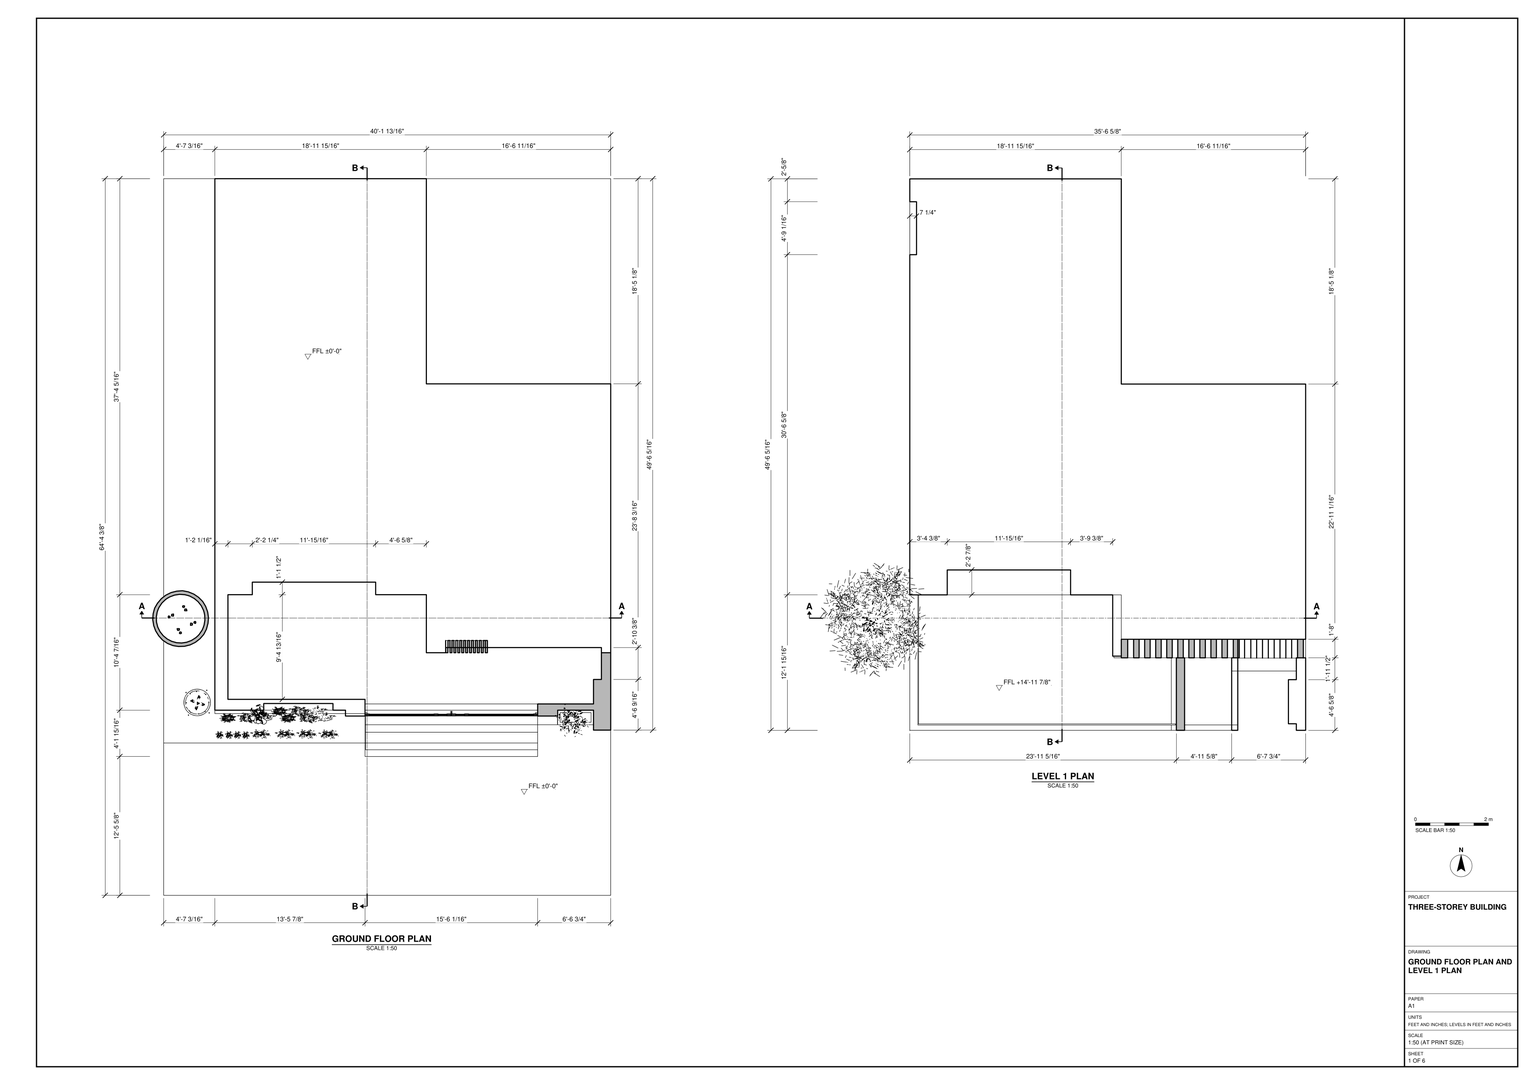
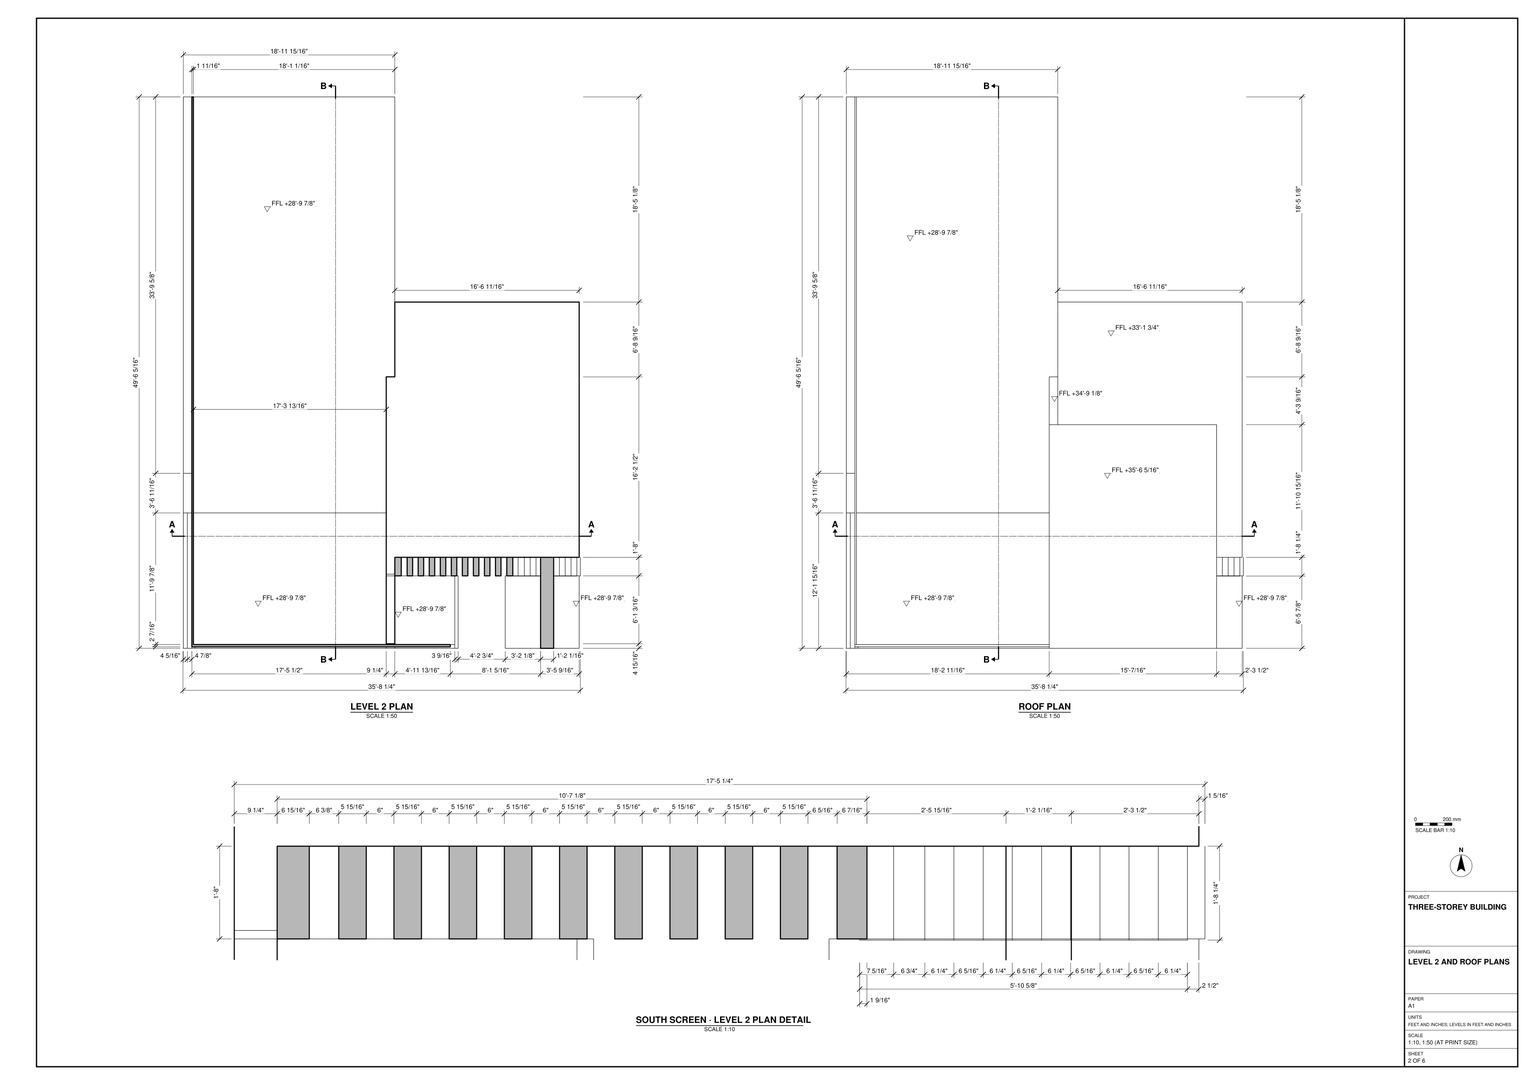
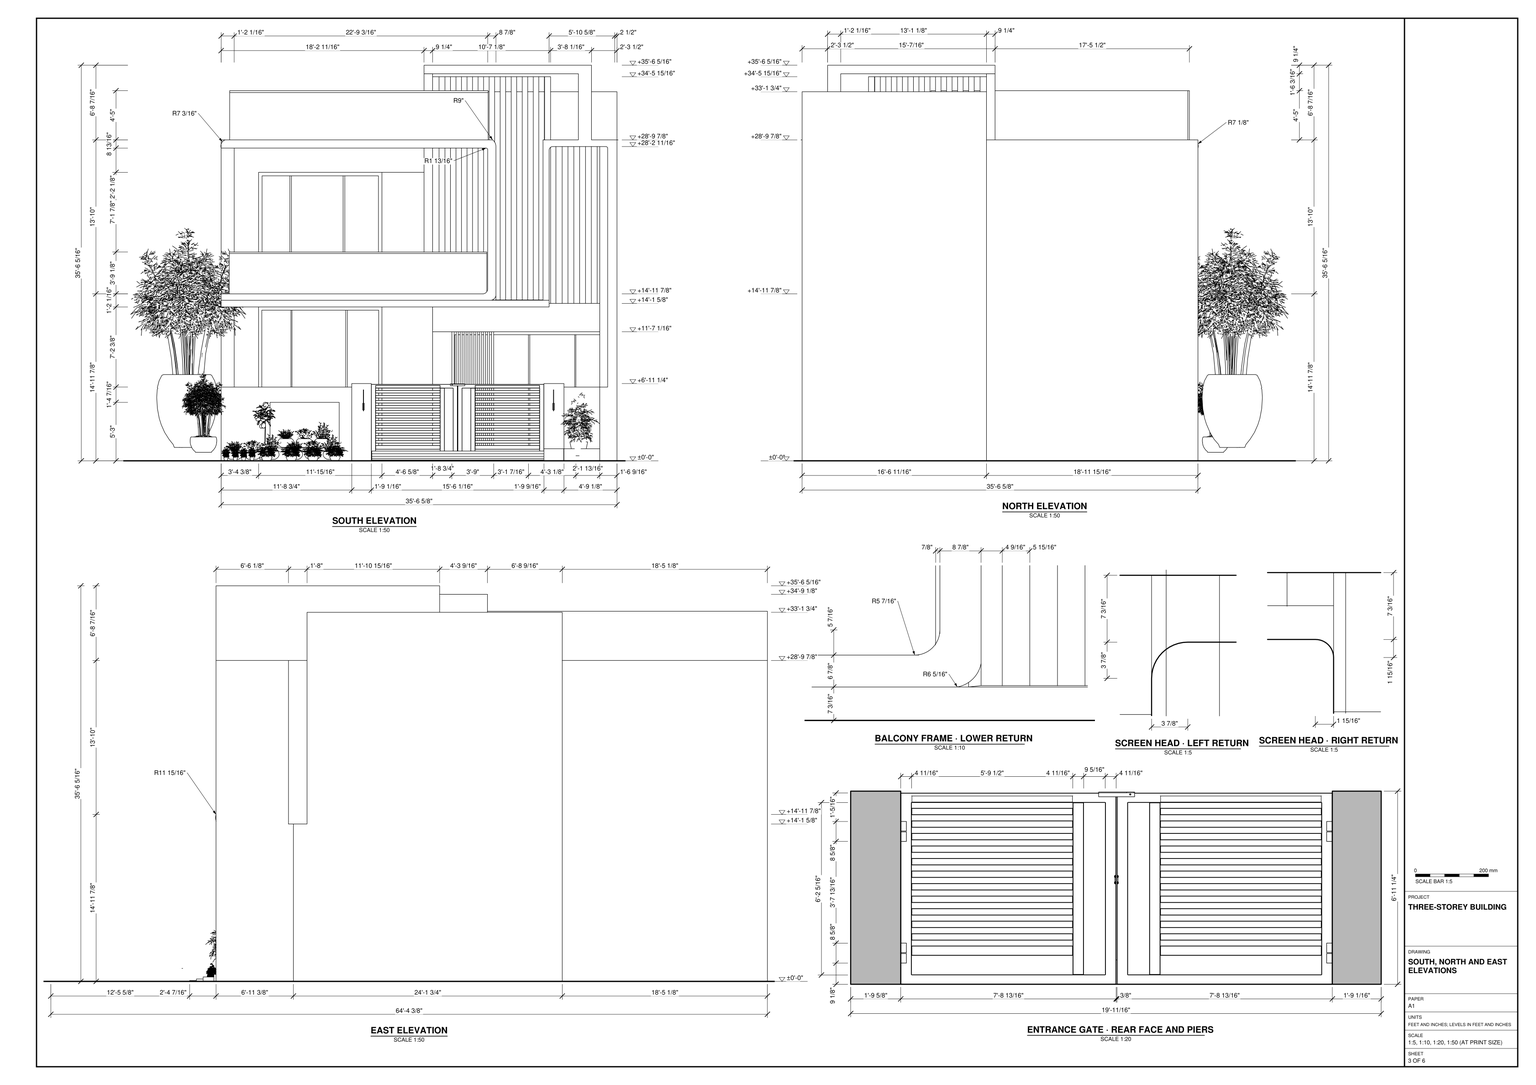
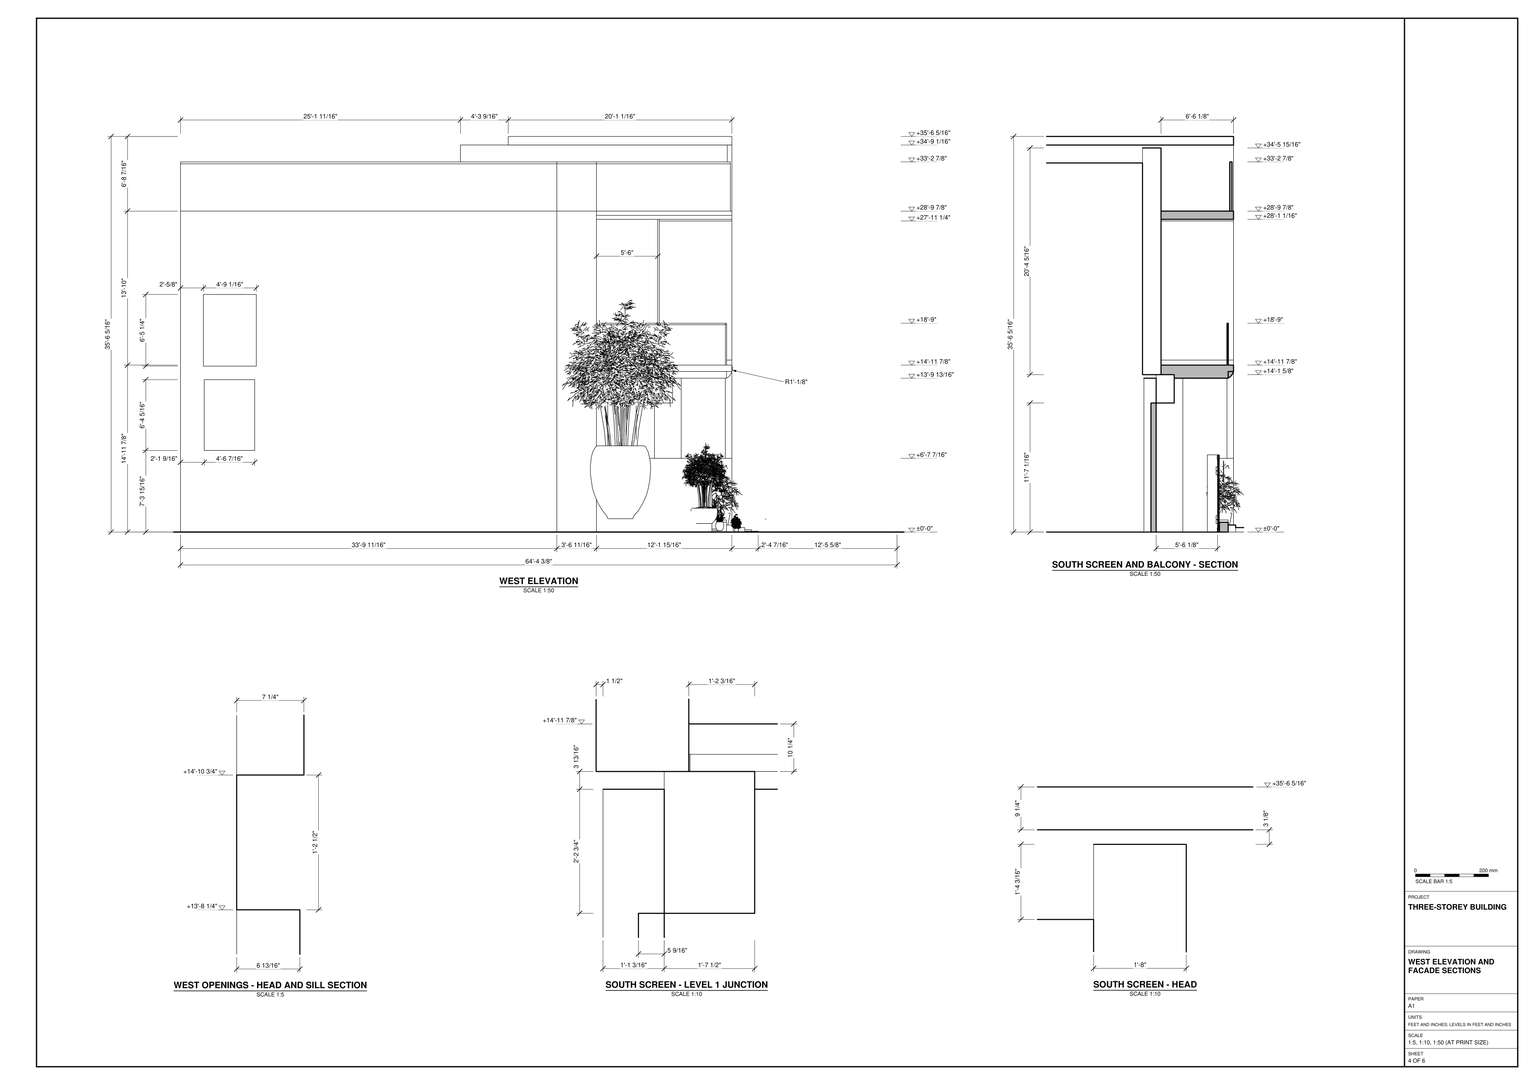
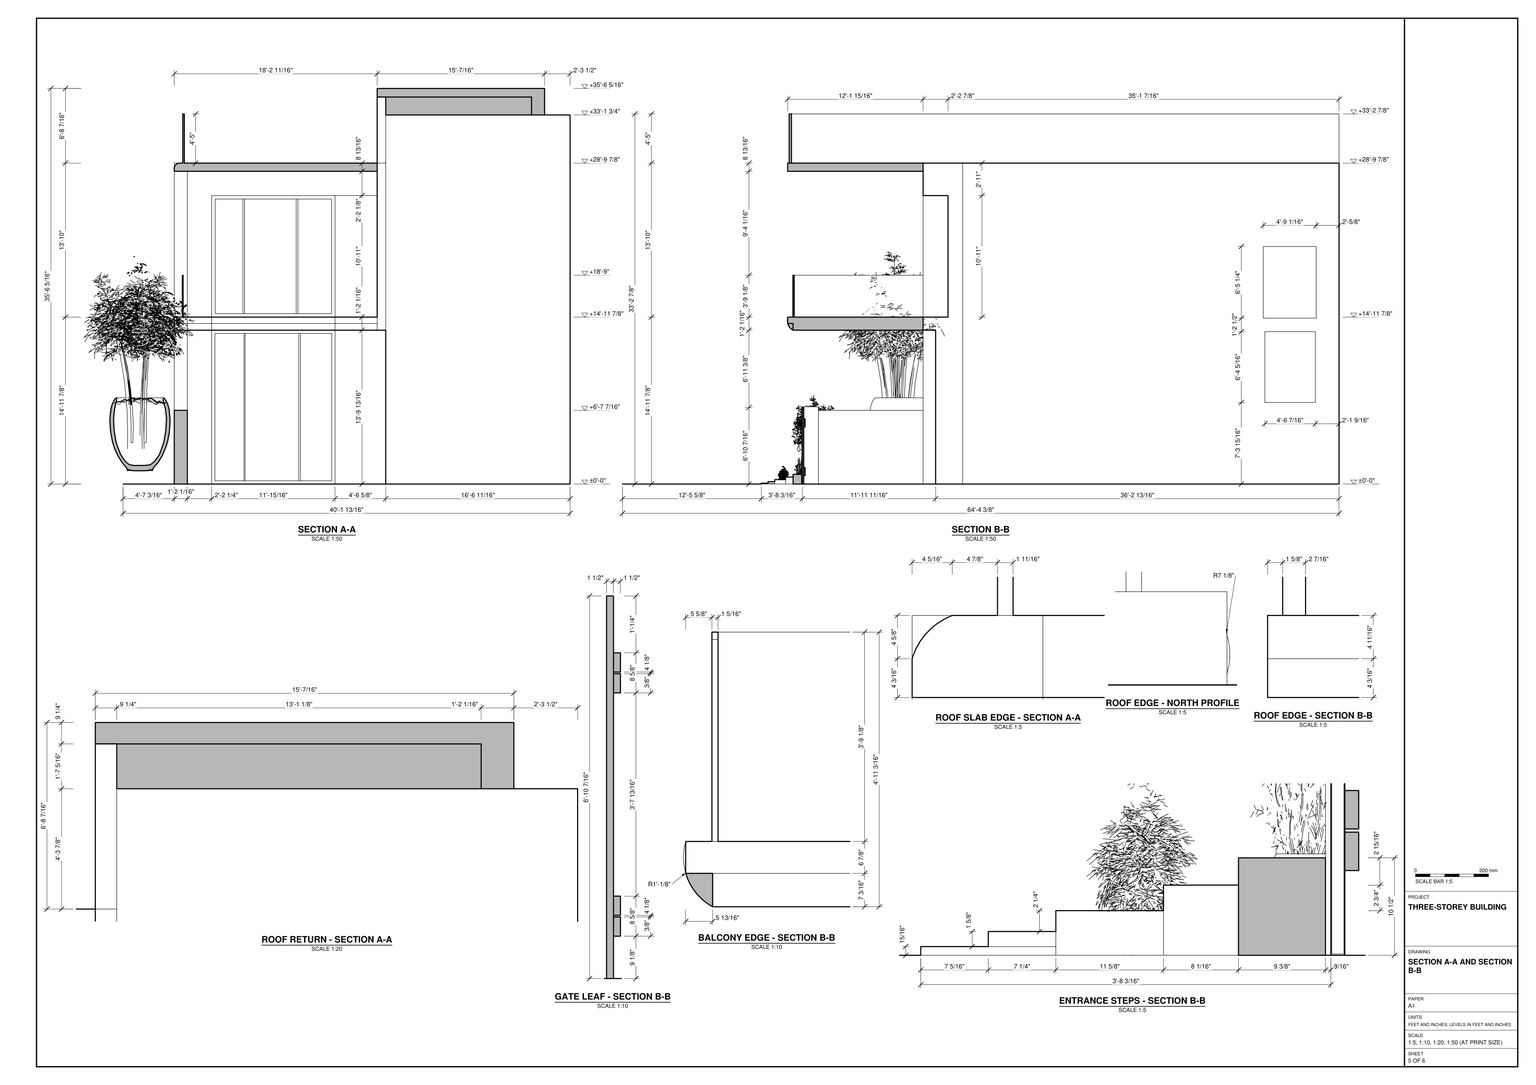
Build the three-storey building and its entrance frontage in SketchUp using task_files/diagram_01.pdf. Work in feet and inches. The complete model shall measure 43'-9 1/8" along X, 64'-4 3/8" along Y and 35'-6 5/16" along Z. Set the ground floor at ±0'-0", Level 1 at +14'-11 7/8" and Level 2 at +28'-9 7/8".

Follow the plans for the stepped footprint, wall thicknesses, openings and slab edges. Use the roof plan and elevations together to locate the changes in roof height. On the south elevation, set the upper glazing behind the balcony parapet, form the rounded returns of the projecting balcony frame, and carry the vertical screen fins up to the raised roof frame. Model the lower glazing, entrance steps, gate leaves and piers, using the rear-face detail for the gate. Include the planting in the positions shown on the frontage plan. Decor and loose items, including plants and lights, may use any suitable library components.

Keep shell elements such as walls, slabs and roof separate as groups or components. Do the same for each furniture or joinery piece shown, and use components for repeated parts such as screen fins. Save one SketchUp model as output_files/three_storey_building_with_a_screened_south_balcony.skp.

# SketchUp Ruby script. Lengths in inches.
U = 1.inch
M = Sketchup.active_model
def pt(a) = Geom::Point3d.new(a.map { |v| v * U })
def face(e, loops, mat)
  f = e.add_face(loops[0].map { |a| pt(a) })
  loops[1..].each { |l| e.add_face(l.map { |a| pt(a) }).erase! }
  f.material = f.back_material = mat if mat
  f
end
# faces: each face lists its corners as indices into pts; further lists are holes
def faces(e, pts, list, mat = nil) = list.each { |f| face(e, (f[0].is_a?(Array) ? f : [f]).map { |l| l.map { |i| pts[i] } }, mat) }
# xy, xz, yz: faces in a plane at the given z, y or x. An outline is a flat list of corners, or four numbers for a rectangle; further outlines are holes
def ring(l) = l.size == 4 ? [[l[0], l[1]], [l[2], l[1]], [l[2], l[3]], [l[0], l[3]]] : l.each_slice(2).to_a
def flat(e, list, mat, &to3) = list.each { |f| face(e, (f[0].is_a?(Array) ? f : [f]).map { |l| ring(l).map { |u, v| to3.(u, v) } }, mat) }
def xy(e, z, list, mat = nil) = flat(e, list, mat) { |x, y| [x, y, z] }
def xz(e, y, list, mat = nil) = flat(e, list, mat) { |x, z| [x, y, z] }
def yz(e, x, list, mat = nil) = flat(e, list, mat) { |y, z| [x, y, z] }
def lines(e, pts, list) = list.each { |a, b| e.add_line(pt(pts[a]), pt(pts[b])) }
# prism: a flat outline (further loops are holes) pulled along v
def prism(e, loops, v, mat = nil)
  f = face(e, loops, mat); d = Geom::Vector3d.new(v.map { |x| x * U })
  f.pushpull(f.normal.samedirection?(d) ? d.length : -d.length)
end
def box(e, o, s, mat = nil) = prism(e, [[o, [o[0] + s[0], o[1], o[2]], [o[0] + s[0], o[1] + s[1], o[2]], [o[0], o[1] + s[1], o[2]]]], [0, 0, s[2]], mat)
def at(x, y, z, deg = 0) = Geom::Transformation.translation(pt([x, y, z])) * Geom::Transformation.rotation(ORIGIN, Z_AXIS, deg.degrees)
def axes(o, x, y, z) = Geom::Transformation.new([*x, 0, *y, 0, *z, 0, *pt(o).to_a, 1])
def part(name) = M.definitions.add(name)
# library, detail: a bought-in or finely detailed component or shape, given as its bounding box
def library(name, o, s) = part(name).tap { |d| box(d.entities, o, s) }
def detail(e, o, s) = box(e.add_group.entities, o, s)
def put(e, d, t, mat = nil) = e.add_instance(d, t).tap { |i| i.material = mat if mat }
def group(e, t, mat = nil) = e.add_group.tap { |g| g.transformation = t; g.material = mat if mat }.entities
root = M.entities
M.materials.add("Material__11").color = [91, 133, 74]
M.materials.add("Material__3").color = [47, 40, 35]
M.materials.add("Material__4").color = [45, 34, 22]
M.materials.add("Material__6").color = [53, 66, 30]
M.materials.add("Niraj_Hair_Dark").color = [109, 109, 109]
M.materials.add("Niraj_Shirt").color = [144, 153, 181]
M.materials.add("[0129_WhiteSmoke]").color = [245, 245, 245]
M.materials.add("[0130_Gainsboro]").color = [220, 220, 220]
M.materials.add("[Asphalt New]").color = [67, 60, 62]
M.materials.add("[Basic Tile]").color = [203, 206, 202]
M.materials.add("[Cladding Siding Tan]").color = [162, 126, 95]
M.materials.add("[Field Square Tile]").color = [217, 201, 169]
M.materials.add("[Grass Dark Green]").color = [106, 157, 55]
M.materials.add("[Translucent Glass Gray]").color = [128, 128, 128]
M.materials["[Translucent Glass Gray]"].alpha = 0.5
M.materials.add("[Wood Floor Parquet]").color = [145, 89, 39]
M.materials.add("[Wood Veneer 01]").color = [120, 70, 37]
M.materials.add("bronze").color = [85, 58, 39]
M.materials.add("light bulb").color = [254, 239, 217]
M.materials.add("wire_1").color = [17, 17, 17]
c1 = library("Slatted double gate",[7.03,-128.55,-3.91],[5.33,99.02,60.06])
c2 = part("Linear wall light")
g1 = group(c2.entities,at(0.6875,0,0.79))
xy(g1,0,[[0,0,0.39,8.27],[[0,8.27,0.39,22.83],[0.04,8.31,0.35,22.8]]])
xy(g1,0.04,[[0.04,8.31,0.35,22.8]],"light bulb")
xy(g1,0.39,[[0,0,0.39,22.83]])
xz(g1,0,[[0,0,0.39,0.39]])
xz(g1,8.31,[[0.04,0,0.35,0.04]])
xz(g1,22.8,[[0.04,0,0.35,0.04]])
xz(g1,22.83,[[0,0,0.39,0.39]])
yz(g1,0,[[0,0,22.83,0.39]])
yz(g1,0.04,[[8.31,0,22.8,0.04]])
yz(g1,0.35,[[8.31,0,22.8,0.04]])
yz(g1,0.39,[[0,0,22.83,0.39]])
g2 = group(c2.entities,at(0,1.18,0))
box(g2,[0,0,0],[1.77,7.09,0.79])
c3 = part("WALL+LIGHT+50")
put(c3.entities,c2,axes([4.75,-2.61,16.86],[1,0,0],[0,0,1],[0,-1,0]),"bronze")
put(c3.entities,c2,axes([209.625,-2.61,16.86],[1,0,0],[0,0,1],[0,-1,0]),"bronze")
c4 = library("plants",[0.18,-0.67,0.63],[15.85,6.49,10.81])
c5 = library("Group\#17",[-156.07,-132.78,403.82],[328.27,343.15,49.73])
c6 = library("Group\#15",[-190.47,-156.43,0],[392.44,392.43,450])
c7 = library("Group\#18",[-224.63,-110.83,370.48],[360.75,278.69,1335.95])
c8 = library("Group\#19",[-170.17,-135.75,412.97],[353.33,352.63,31.3])
c9 = library("Group\#14",[-390.42,-321.9,981.25],[712.69,695.89,825.3])
c10 = part("Potted tree")
p = [[391.42,322.9,0],[390.42,321.9,0],[391.42,321.9,0]]
lines(c10.entities,p,[[0,1],[1,2],[2,0]])
put(c10.entities,c5,at(390.42,321.9,0),"Material__3")
put(c10.entities,c6,at(390.42,321.9,0))
put(c10.entities,c7,at(390.42,321.9,0),"Material__4")
g3 = group(c10.entities,at(390.42,321.9,0),"wire_1")
xy(g3,2.45,[[-59.6,-46.28,-36.375,-34.93,-11.68,-29.34,15.46,-33.14,46.57,-25.27,76.1,-6.18,100.39,22.24,98.66,53.87,95.77,65.28,88.08,79.53,87.97,84.15,87.1,85.66,83.13,88.01,74.2,100.3,66.09,109.96,37.49,121.54,1.58,115.97,-27.44,104.75,-47.08,82.45,-56.52,55.13,-74.46,34.57,-97.22,27.4375,-113.62,-7.42,-100.95,-13.99,-91.64,-16.18,-96.41,-18.55,-93.97,-22.4375,-89.59,-19.73,-91.56,-27.7,-91.98,-39.95]],"wire_1")
put(c10.entities,c8,at(390.42,321.9,0),"Material__3")
put(c10.entities,c9,at(390.42,321.9,0),"Material__6")
c11 = library("Group\#24",[-51.25,-16.26,0.11],[32.43,32.44,25.32])
c12 = library("Group\#29",[-68.4,-38.23,21.61],[71.82,69.27,94.54])
c13 = library("Group\#31",[0,0,0],[126.13,128.05,229.04])
c14 = library("Group\#32",[0,23.8125,0],[126.13,128.06,238.18])
c15 = part("BAMBOO+PLANTS+18")
p = [[0,0,0],[1,0,0],[1,1,0]]
lines(c15.entities,p,[[0,1],[1,2],[2,0]])
put(c15.entities,c11,axes([-463.4375,32.99,-14],[0.36589,0,0],[0,0.16797,0],[0,0,0.16797]))
put(c15.entities,c12,axes([-463.4375,32.99,-14],[0.36589,0,0],[0,0.16797,0],[0,0,0.16797]),"Material__11")
put(c15.entities,c13,axes([-568.04,42.06,-4.9],[0.38,0,0],[0,0.38,0],[0,0,0.38]))
put(c15.entities,c11,axes([-119.36,48.1875,-8.59],[0.59,0,0],[0,0.59,0],[0,0,0.59]))
put(c15.entities,c12,axes([-119.36,48.1875,-8.59],[0.59,0,0],[0,0.59,0],[0,0,0.59]),"Material__11")
put(c15.entities,c14,at(-623.98,68,0.35))
put(c15.entities,c11,axes([-436.93,32.99,-14],[0.36589,0,0],[0,0.16797,0],[0,0,0.16797]))
put(c15.entities,c12,axes([-436.93,32.99,-14],[0.36589,0,0],[0,0.16797,0],[0,0,0.16797]),"Material__11")
put(c15.entities,c12,axes([-413.65,32.99,-14],[0.36589,0,0],[0,0.16797,0],[0,0,0.16797]),"Material__11")
put(c15.entities,c11,axes([-413.65,32.99,-14],[0.36589,0,0],[0,0.16797,0],[0,0,0.16797]))
put(c15.entities,c11,axes([-390,32.72,-13.61],[0.36589,0,0],[0,0.16797,0],[0,0,0.16797]))
put(c15.entities,c12,axes([-390,32.72,-13.61],[0.36589,0,0],[0,0.16797,0],[0,0,0.16797]),"Material__11")
put(c15.entities,c12,axes([-505.28,31.89,-14],[0.14036,0,0],[0,0.14036,0],[0,0,0.14036]),"Material__11")
put(c15.entities,c11,axes([-487.28,31.66,-13.67],[0.14036,0,0],[0,0.14036,0],[0,0,0.14036]))
put(c15.entities,c12,axes([-487.28,31.66,-13.67],[0.14036,0,0],[0,0.14036,0],[0,0,0.14036]),"Material__11")
put(c15.entities,c11,axes([-505.28,31.89,-14],[0.14036,0,0],[0,0.14036,0],[0,0,0.14036]))
put(c15.entities,c11,axes([-515.45,31.89,-14],[0.14036,0,0],[0,0.14036,0],[0,0,0.14036]))
put(c15.entities,c12,axes([-515.45,31.89,-14],[0.14036,0,0],[0,0.14036,0],[0,0,0.14036]),"Material__11")
put(c15.entities,c11,axes([-496.35,31.89,-14],[0.14036,0,0],[0,0.14036,0],[0,0,0.14036]))
put(c15.entities,c12,axes([-496.35,31.89,-14],[0.14036,0,0],[0,0.14036,0],[0,0,0.14036]),"Material__11")
c16 = library("Group\#2",[0,0,0],[149.58,6.3125,301.125])
c17 = library("Group\#3",[0,0,0],[149.58,6.3125,301.125])
c18 = library("Group\#1",[0,0,0],[78.59,6.3125,301.125])
xy(root,0,[[463.28,178.07,481.82,178.07,481.82,261.48,471.78,261.48,471.78,232.66,463.28,232.66,463.28,206.28,403.07,206.28,403.07,193.25,424.67,193.25,424.67,199.56,463.28,199.56],[217.61,183.87,424.39,193.25],[424.39,183.87,424.67,193.25],[[424.67,183.87,463.28,199.56],[427.29,186.49,460.66,196.9375]],[427.29,186.49,460.66,196.9375],
  [217.61,193.25,403.07,193.25,403.07,199.56,217.02,199.56,217.02,195.87,217.61,195.87],[55.17,195.87,195.95,199.56],[217.02,199.56,403.07,206.28],[217.02,206.28,463.28,206.28,463.28,232.66,471.78,232.66,471.78,267.04,303.9,267.04,303.9,261.48,283.13,261.48,283.13,324.02,228.49,324.02,228.49,337.52,95.53,337.52,95.53,324.02,69.26,324.02,69.26,211.22,217.02,211.22],[283.13,551.23,481.82,772.36]])
xy(root,0,[[0,0,481.82,0,481.82,178.07,463.28,178.07,463.28,183.87,403.07,183.87,403.07,149.62,217.02,149.62,217.02,164.18,0,164.18]],"[Basic Tile]")
xy(root,0,[[195.95,193.25,217.02,195.87],[195.95,195.87,217.02,195.87,217.02,211.22,69.26,211.22,69.26,324.02,95.53,324.02,95.53,337.52,228.49,337.52,228.49,324.02,283.13,324.02,283.13,261.48,303.9,261.48,303.9,267.04,471.78,267.04,471.78,261.48,481.82,261.48,481.82,551.23,283.13,551.23,283.13,772.36,55.17,772.36,55.17,199.56,195.95,199.56]],"[Field Square Tile]")
xy(root,0,[[0,164.18,217.02,164.18,217.02,193.25,195.95,193.25,195.95,195.87,55.17,195.87,55.17,772.36,0,772.36],[217.02,164.18,217.61,183.87],[217.02,183.87,217.61,193.25],[217.02,193.25,217.61,195.87]],"[Grass Dark Green]")
xy(root,0.9375,[[217.02,149.62,403.07,149.62,403.07,156.9,217.61,156.9,217.61,164.18,217.02,164.18]],"[Field Square Tile]")
xy(root,2.5625,[[217.61,156.9,403.07,164.18]],"[Field Square Tile]")
xy(root,4.8125,[[217.61,164.18,403.07,175.79]],"[Field Square Tile]")
xy(root,7.5625,[[217.61,175.79,403.07,183.87]],"[Field Square Tile]")
xy(root,10.5,[[217.61,183.87,403.07,193.25]],"[Field Square Tile]")
xy(root,13,[[403.07,183.87,424.39,193.25],[[424.67,183.87,463.28,199.56],[427.29,186.49,460.66,196.9375]]],"[Asphalt New]")
xy(root,13.87,[[107.84,199.56,182.46,206.75]])
xy(root,62.99,[[107.84,199.56,182.46,206.75]])
xy(root,79.4375,[[463.28,178.07,471.78,185.12],[463.28,185.12,471.78,199.56],[55.17,199.56,195.95,199.56,195.95,211.22,69.26,211.22,69.26,324.02,55.17,324.02],[424.67,199.56,458.84,199.56,458.84,203.37,463.28,203.37,463.28,206.28,424.67,206.28],[458.84,199.56,463.28,203.37]])
xy(root,83.25,[[195.95,193.25,217.02,211.22],[403.07,193.25,424.67,206.28]])
xy(root,87.94,[[55.17,692.36,61.99,746.8]],"[0129_WhiteSmoke]")
xy(root,139.07,[[465.71,241.98,471.78,267.04]])
xy(root,139.07,[[283.13,241.98,303.9,261.48],[303.9,241.98,465.71,267.04]],"[Asphalt New]")
xy(root,164.25,[[55.17,692.36,61.99,746.8]],"[0129_WhiteSmoke]")
xy(root,165.8125,[[95.53,324.02,228.49,337.52]])
xy(root,165.8125,[[55.17,183.87,55.17,324.02,283.13,324.02,283.13,241.98,408.69,241.98,408.69,183.87]],"[Field Square Tile]")
xy(root,169.64,[[283.13,241.98,351.34,256.18],[408.69,241.98,471.78,241.98,471.78,256.18,481.82,256.18,481.82,276.16,283.13,276.16,283.13,256.18,408.69,256.18],[351.34,241.98,408.69,256.18]])
xy(root,173.02,[[55.17,178.06,346.23,178.07],[55.17,178.07,346.23,183.87],[346.23,178.07,348.65,183.87],[348.65,178.07,408.69,183.87],[346.23,183.87,348.65,197.12],
  [275.14,224.23,283.13,256.18]])
xy(root,173.33,[[351.34,178.07,402.09,256.18]])
xy(root,178.78,[[55.17,690.64,62.42,747.7]],"[0129_WhiteSmoke]")
xy(root,179.89,[[55.17,178.06,337.03,178.06,337.03,183.71,63.89,183.71,63.89,324.02,55.17,324.02],[337.03,183.71,341.53,185.04],[64.7,185.04,337.03,185.04,337.03,256.18,275.14,256.18,275.14,258,273.88,258,273.88,324.02,64.7,324.02],[275.14,256.18,283.13,258],[95.53,324.02,228.49,350.9]])
xy(root,225.02,[[63.89,183.71,341.53,185.04],[63.89,185.04,64.7,324.02]],"Niraj_Hair_Dark")
xy(root,256.03,[[55.17,690.64,62.42,747.7]],"[0129_WhiteSmoke]")
xy(root,310.89,[[95.53,324.02,228.49,350.9]])
xy(root,337.03,[[273.88,256.18,283.13,258]])
xy(root,337.03,[[55.17,178.06,55.17,324.02,69.26,324.02,69.26,206.96,340.65,206.96,340.65,178.06]],"[Field Square Tile]")
xy(root,337.03,[[69.26,206.96,256.26,324.02],[256.26,206.96,256.26,324.02,273.88,324.02,273.88,256.18,340.65,256.18,340.65,206.96]],"[Wood Floor Parquet]")
xy(root,338.67,[[412.59,178.07,469.83,185.12]])
xy(root,342.31,[[463.28,185.12,471.78,232.66]])
xy(root,345.875,[[59.49,178.06,64.375,324.02],[64.375,178.06,67.74,179.68],[67.74,178.06,273.88,179.68],[273.88,178.06,283.13,179.68],[283.13,178.06,347.76,178.06,347.76,182.15,342.94,182.15,342.94,179.68,283.13,179.68],
  [64.375,179.68,342.94,182.15],[66.05,182.15,273.88,324.02],[273.88,182.15,283.13,183],[283.13,182.15,347.76,256.18],[273.88,183,283.13,256.18],
  [64.375,324.02,66.05,772.36],[66.05,324.02,273.88,324.02,273.88,470.65,283.13,470.65,283.13,772.36,66.05,772.36],[55.17,366.7,64.375,772.36]])
xy(root,345.875,[[55.17,324.02,64.375,366.7]],"Niraj_Shirt")
xy(root,345.875,[[402.09,178.07,440.24,256.18],[454.32,178.07,481.82,256.18],[440.24,256.18,454.32,276.16]],"[0129_WhiteSmoke]")
xy(root,397.75,[[283.13,276.16,440.24,276.16,440.24,419.1,454.32,419.1,454.32,276.16,481.82,276.16,481.82,551.23,283.13,551.23]])
xy(root,397.75,[[440.24,276.16,454.32,419.1]],"[0129_WhiteSmoke]")
xy(root,398.875,[[64.375,179.68,342.94,182.15],[64.375,182.15,66.05,772.36]],"Niraj_Hair_Dark")
xy(root,417.08,[[283.13,178.07,283.13,183,273.88,183,273.88,419.1,440.24,419.1,440.24,178.07]],"[0129_WhiteSmoke]")
xy(root,417.125,[[273.88,178.07,283.13,183],[273.88,183,283.13,470.65]])
xy(root,426.3125,[[273.88,178.07,454.32,419.1]],"[0129_WhiteSmoke]")
xz(root,149.62,[[217.02,0,403.07,0.9375]],"[Field Square Tile]")
xz(root,156.9,[[217.61,0.9375,403.07,2.5625]],"[Field Square Tile]")
xz(root,164.18,[[217.02,0,217.61,0.9375]])
xz(root,164.18,[[217.61,2.5625,403.07,4.8125]],"[Field Square Tile]")
xz(root,175.79,[[217.61,4.8125,403.07,7.5625]],"[Field Square Tile]")
xz(root,178.06,[[55.17,173.02,346.23,173.02,346.85,173.16,347.46,173.37,348.04,173.64,348.59,173.97,348.65,174.01,349.11,174.35,349.58,174.78,350.01,175.25,350.39,175.77,350.71,176.32,350.98,176.9,351.19,177.5,351.34,178.125,351.34,338.7,351.3125,339.39,351.23,340.08,351.1,340.76,350.92,341.43,350.68,342.08,350.4,342.71,350.0625,343.32,349.68,343.9,349.26,344.44,348.8,344.96,348.3,345.4375,347.76,345.875,59.49,345.875,58.67,345.5,57.9,345.03,57.2,344.46,56.58,343.8125,56.04,343.09,55.59,342.31,55.25,341.47,55.17,341.21,55.17,337.03,340.65,337.03,340.89,337.02,341.12,336.97,341.34,336.9,341.56,336.79,341.75,336.66,341.93,336.5,342.09,336.33,342.22,336.13,342.32,335.92,342.4,335.69,342.45,335.46,342.46,335.23,342.46,185.33,342.41,184.62,342.28,183.92,342.05,183.25,341.73,182.61,341.34,182.02,340.87,181.48,340.33,181.01,339.74,180.62,339.11,180.31,338.43,180.08,337.74,179.9375,337.03,179.89,55.17,179.89],[55.17,337.03,55.17,341.21,55.01,340.6,54.88,339.71,54.87,338.81,54.96,337.91]])
xz(root,178.07,[[463.28,0,481.82,0,481.82,345.875,454.32,345.875,454.32,426.3125,273.88,426.3125,273.88,417.125,283.13,417.125,283.13,417.08,440.24,417.08,440.24,345.875,402.09,345.875,402.09,173.33,351.34,173.33,348.65,173.02,408.69,173.02,408.69,334.77,408.73,335.28,408.83,335.78,408.99,336.26,409.22,336.72,409.5,337.14,409.83,337.53,410.22,337.86,410.64,338.15,411.1,338.37,411.58,338.54,412.08,338.64,412.59,338.67,469.83,338.67,470.08,338.65,470.33,338.6,470.57,338.52,470.8,338.41,471.01,338.27,471.21,338.1,471.375,337.91,471.52,337.69,471.63,337.47,471.71,337.22,471.76,336.97,471.78,336.72,471.78,79.4375,463.28,79.4375]])
xz(root,179.68,[[64.375,396.83,342.94,398.875]],"Niraj_Hair_Dark")
xz(root,179.68,[[64.375,345.875,342.94,396.83]],"[Translucent Glass Gray]")
xz(root,182.15,[[66.05,345.875,342.94,398.875]],"[Translucent Glass Gray]")
xz(root,183,[[273.88,345.875,283.13,417.08],[273.88,417.08,283.13,417.125]])
xz(root,183.71,[[63.89,223.42,341.53,225.02]],"Niraj_Hair_Dark")
xz(root,183.71,[[63.89,179.89,341.53,223.42]],"[Translucent Glass Gray]")
xz(root,183.87,[[217.61,0,403.07,7.5625],[55.17,165.8125,408.69,173.02]])
xz(root,183.87,[[403.07,0,424.39,13],[424.67,0,463.28,13]],"[Asphalt New]")
xz(root,183.87,[[217.61,7.5625,403.07,10.5]],"[Field Square Tile]")
xz(root,185.04,[[63.89,179.89,64.7,225.02]])
xz(root,185.04,[[64.7,179.89,341.53,225.02]],"[Translucent Glass Gray]")
xz(root,185.12,[[463.28,79.4375,471.78,79.4375,471.78,336.72,471.76,336.97,471.71,337.22,471.63,337.47,471.52,337.69,471.375,337.91,471.21,338.1,471.01,338.27,470.8,338.41,470.57,338.52,470.33,338.6,470.08,338.65,469.83,338.67,463.28,338.67],[471.78,336.72,471.78,342.31,463.28,342.31,463.28,338.67,469.83,338.67,470.08,338.65,470.33,338.6,470.57,338.52,470.8,338.41,471.01,338.27,471.21,338.1,471.375,337.91,471.52,337.69,471.63,337.47,471.71,337.22,471.76,336.97]])
xz(root,186.49,[[427.29,0,460.66,13]])
xz(root,193.25,[[195.95,0,217.02,83.25],[217.61,0,403.07,10.5],[403.07,0,424.39,13],[424.39,0,424.67,0,424.67,83.25,403.07,83.25,403.07,13,424.39,13]])
xz(root,196.9375,[[427.29,0,460.66,13]],"[Asphalt New]")
xz(root,197.12,[[346.23,173.02,348.65,173.02,348.65,174.01,348.59,173.97,348.04,173.64,347.46,173.37,346.85,173.16],[348.65,173.02,351.34,173.02,351.34,173.33],[348.65,173.02,351.34,173.33,351.34,178.125,351.19,177.5,350.98,176.9,350.71,176.32,350.39,175.77,350.01,175.25,349.58,174.78,349.11,174.35,348.65,174.01],[348.65,174.01,349.11,174.35,349.58,174.78,350.01,175.25,350.39,175.77,350.71,176.32,350.98,176.9,351.19,177.5,351.34,178.125,348.65,178.125]])
xz(root,199.56,[[[55.17,0,195.95,79.4375],[107.84,13.87,182.46,62.99]],[424.67,0,463.28,13],[424.67,13,463.28,79.4375]])
xz(root,206.28,[[403.07,0,403.07,83.25,424.67,83.25,424.67,79.4375,463.28,79.4375,463.28,0]])
xz(root,206.75,[[107.84,13.87,182.46,62.99]])
xz(root,211.22,[[69.26,0,217.02,79.4375],[195.95,79.4375,217.02,83.25]])
xz(root,232.66,[[463.28,0,471.78,342.31]])
xz(root,241.98,[[283.13,165.8125,408.69,169.64]])
xz(root,241.98,[[283.13,139.07,471.78,139.07,471.78,169.64,408.69,169.64,408.69,165.8125,283.13,165.8125]],"[Asphalt New]")
xz(root,256.18,[[283.13,169.64,283.13,179.89,342.46,179.89,342.46,337.03,283.13,337.03,283.13,345.875,347.76,345.875,348.3,345.4375,348.8,344.96,349.26,344.44,349.68,343.9,350.0625,343.32,350.4,342.71,350.68,342.08,350.92,341.43,351.1,340.76,351.23,340.08,351.3125,339.39,351.34,338.7,351.34,169.64],[351.34,169.64,351.34,173.33,402.09,173.33,402.09,330.87,408.69,330.87,408.69,169.64],[471.78,169.64,481.82,330.87],[275.14,173.02,283.13,179.89],[337.03,179.89,337.74,179.9375,338.43,180.08,339.11,180.31,339.74,180.62,340.33,181.01,340.87,181.48,341.34,182.02,341.73,182.61,342.05,183.25,342.28,183.92,342.41,184.62,342.46,185.33,342.46,179.89],
  [471.78,330.87,481.82,345.875],[342.46,335.23,342.45,335.46,342.4,335.69,342.32,335.92,342.22,336.13,342.09,336.33,341.93,336.5,341.75,336.66,341.56,336.79,341.34,336.9,341.12,336.97,340.89,337.02,340.65,337.03,342.46,337.03],[273.88,337.03,283.13,345.875]])
xz(root,256.18,[[402.09,330.87,408.69,345.875]],"[0129_WhiteSmoke]")
xz(root,258,[[273.88,179.89,283.13,337.03]])
xz(root,261.48,[[471.78,0,481.82,139.07]])
xz(root,261.48,[[283.13,0,303.9,139.07]],"[Asphalt New]")
xz(root,267.04,[[303.9,0,386.39,0,386.39,3.15,307.06,3.15,307.06,135.91,468.625,135.91,468.625,3.15,387.84,3.15,387.84,0,471.78,0,471.78,139.07,303.9,139.07],[386.39,0,387.84,3.15],[386.39,3.15,387.84,135.91],[436.29,3.15,437.49,135.91]],"[Asphalt New]")
xz(root,267.04,[[307.06,3.15,386.39,135.91],[387.84,3.15,436.29,135.91],[437.49,3.15,468.625,135.91]],"[Translucent Glass Gray]")
xz(root,276.16,[[440.24,345.875,454.32,397.75]],"[0129_WhiteSmoke]")
xz(root,276.16,[[410.27,345.875,440.24,397.75],[454.32,345.875,481.82,397.75]],"[Translucent Glass Gray]")
xz(root,276.16,[[283.13,169.64,481.82,169.64,481.82,345.875,410.27,345.875,410.27,397.75,283.13,397.75]],"[Wood Floor Parquet]")
xz(root,324.02,[[55.17,165.8125,69.26,173.02],[69.26,165.8125,95.53,173.02],[95.53,165.8125,228.49,173.02],[228.49,165.8125,273.88,173.02],[55.17,173.02,55.17,179.89,63.89,179.89,63.89,225.02,64.7,225.02,64.7,179.89,69.26,179.89,69.26,173.02],
  [69.26,173.02,95.53,179.89],[95.53,173.02,228.49,179.89],[228.49,173.02,273.88,179.89],[55.17,337.03,55.17,341.21,55.25,341.47,55.59,342.31,56.04,343.09,56.58,343.8125,57.2,344.46,57.9,345.03,58.67,345.5,59.49,345.875,69.26,345.875,69.26,337.03],[69.26,337.03,95.53,345.875],
  [95.53,337.03,228.49,345.875],[228.49,337.03,273.88,345.875],[55.17,341.21,55.17,345.875,59.49,345.875,58.67,345.5,57.9,345.03,57.2,344.46,56.58,343.8125,56.04,343.09,55.59,342.31,55.25,341.47]])
xz(root,324.02,[[55.17,79.4375,69.26,165.8125],[55.17,179.89,63.89,179.89,63.89,225.02,64.7,225.02,64.7,179.89,69.26,179.89,69.26,337.03,55.17,337.03]],"Niraj_Shirt")
xz(root,324.02,[[69.26,0,95.53,165.8125],[69.26,179.89,95.53,179.89,95.53,310.89,273.88,310.89,273.88,337.03,69.26,337.03]],"[Asphalt New]")
xz(root,324.02,[[228.49,0,283.13,165.8125],[228.49,179.89,273.88,310.89]],"[Cladding Siding Tan]")
xz(root,337.52,[[[95.53,0,228.49,165.8125],[99.02,3.49,225,162.32]],[130.35,3.49,131.54,162.32],[189.42,3.49,191.24,162.32]],"[Asphalt New]")
xz(root,337.52,[[99.02,3.49,130.35,162.32],[131.54,3.49,189.42,162.32],[191.24,3.49,225,162.32]],"[Translucent Glass Gray]")
xz(root,350.9,[[[95.53,179.89,228.49,310.89],[99.3,183.66,224.72,307.12]],[129.23,183.66,130.94,307.12],[186.62,183.66,188.46,307.12]],"[Asphalt New]")
xz(root,350.9,[[99.3,183.66,129.23,307.12],[130.94,183.66,186.62,307.12],[188.46,183.66,224.72,307.12]],"[Translucent Glass Gray]")
xz(root,419.1,[[440.24,397.75,440.24,417.08,273.88,417.08,273.88,426.3125,454.32,426.3125,454.32,397.75]],"[0129_WhiteSmoke]")
xz(root,470.65,[[273.88,345.875,283.13,417.125]])
xz(root,551.23,[[283.13,0,481.82,397.75]],"[Basic Tile]")
xz(root,690.64,[[55.17,178.78,62.42,256.03]],"[0129_WhiteSmoke]")
xz(root,692.36,[[55.17,87.94,61.99,164.25]],"[0129_WhiteSmoke]")
xz(root,746.8,[[55.17,87.94,61.99,164.25]],"[0129_WhiteSmoke]")
xz(root,747.7,[[55.17,178.78,62.42,256.03]],"[0129_WhiteSmoke]")
xz(root,772.36,[[64.375,345.875,66.05,398.875]])
xz(root,772.36,[[55.17,0,283.13,345.875]],"[Basic Tile]")
yz(root,55.17,[[199.56,0,324.02,79.4375],[183.87,165.8125,182.71,166.54,181.63,167.39,180.66,168.36,179.8,169.43,179.07,170.59,178.48,171.83,178.07,173.02,183.87,173.02],[183.87,165.8125,324.02,173.02],[178.06,173.02,178.06,173.04,178.07,173.02],[178.07,173.02,178.06,173.04,178.06,179.89,324.02,179.89,324.02,173.02],
  [178.06,173.04,178.03,173.12,177.73,174.46,177.58,175.82,177.58,177.19,177.74,178.56,178.06,179.89],[178.06,337.03,324.02,341.21]])
yz(root,55.17,[[324.02,0,366.7,345.875]],"Niraj_Shirt")
yz(root,55.17,[[[366.7,0,772.36,345.875],[690.64,178.78,747.7,256.03],[692.36,87.94,746.8,164.25]]],"[0129_WhiteSmoke]")
yz(root,61.99,[[692.36,87.94,746.8,164.25]],"[Translucent Glass Gray]")
yz(root,62.42,[[690.64,178.78,747.7,256.03]],"[Translucent Glass Gray]")
yz(root,63.89,[[183.71,179.89,185.04,223.42],[183.71,223.42,185.04,225.02],[185.04,223.42,324.02,225.02]],"Niraj_Hair_Dark")
yz(root,63.89,[[185.04,179.89,324.02,223.42]],"[Translucent Glass Gray]")
yz(root,64.375,[[179.68,396.83,324.02,398.875],[324.02,396.83,366.7,398.875],[366.7,396.83,772.36,398.875]],"Niraj_Hair_Dark")
yz(root,64.375,[[324.02,345.875,366.7,396.83]],"Niraj_Shirt")
yz(root,64.375,[[366.7,345.875,772.36,396.83]],"[0129_WhiteSmoke]")
yz(root,64.375,[[179.68,345.875,324.02,396.83]],"[Translucent Glass Gray]")
yz(root,64.7,[[185.04,179.89,324.02,225.02]],"[Translucent Glass Gray]")
yz(root,66.05,[[182.15,345.875,772.36,398.875]],"[Translucent Glass Gray]")
yz(root,69.26,[[211.22,0,324.02,79.4375]])
yz(root,95.53,[[324.02,0,337.52,165.8125],[324.02,179.89,350.9,310.89]])
yz(root,107.84,[[199.56,13.87,206.75,62.99]])
yz(root,182.46,[[199.56,13.87,206.75,62.99]])
yz(root,195.95,[[193.25,0,193.25,83.25,211.22,83.25,211.22,79.4375,199.56,79.4375,199.56,0]])
yz(root,217.02,[[149.62,0,164.18,0.9375],[193.25,0,211.22,83.25]])
yz(root,217.61,[[164.18,0,175.79,4.8125],[175.79,0,183.87,7.5625],[183.87,0,193.25,10.5],[156.9,0.9375,164.18,2.5625]])
yz(root,228.49,[[324.02,0,337.52,165.8125],[324.02,179.89,350.9,310.89]])
yz(root,273.88,[[258,179.89,324.02,337.03],[256.18,337.03,324.02,345.875],[183,345.875,183,417.08,419.1,417.08,419.1,417.125,470.65,417.125,470.65,345.875],[183,417.08,419.1,417.125]])
yz(root,273.88,[[178.07,417.125,419.1,426.3125]],"[0129_WhiteSmoke]")
yz(root,283.13,[[551.23,0,772.36,345.875],[256.18,169.64,276.16,169.64,276.16,397.75,183,397.75,183,345.875,256.18,345.875,256.18,337.03,258,337.03,258,179.89,256.18,179.89],[470.65,345.875,551.23,397.75],[183,397.75,470.65,417.125],[178.07,417.08,183,417.125]])
yz(root,283.13,[[261.48,0,281.1875,139.07],[311.89,0,324.02,139.07],[241.98,139.07,324.02,165.8125]],"[Asphalt New]")
yz(root,283.13,[[281.1875,0,311.89,139.07]],"[Translucent Glass Gray]")
yz(root,303.9,[[261.48,0,267.04,139.07]])
yz(root,341.53,[[183.71,179.89,185.04,225.02]])
yz(root,342.46,[[178.06,185.33,256.18,335.23]],"[Wood Floor Parquet]")
yz(root,342.94,[[179.68,345.875,182.15,398.875]])
yz(root,351.34,[[197.12,173.33,256.18,173.33,256.18,338.7,178.06,338.7,178.06,178.125,197.12,178.125],[183.52,173.33,197.12,178.125]])
yz(root,402.09,[[178.07,173.33,256.18,345.875]],"[0130_Gainsboro]")
yz(root,403.07,[[149.62,0,156.9,0.9375],[156.9,0,164.18,2.5625],[164.18,0,175.79,4.8125],[175.79,0,183.87,7.5625],[193.25,0,206.28,83.25],
  [183.87,10.5,193.25,13]])
yz(root,408.69,[[183.87,165.8125,183.87,173.02,178.07,173.02,178.48,171.83,179.07,170.59,179.8,169.43,180.66,168.36,181.63,167.39,182.71,166.54],[183.87,165.8125,241.98,169.64],[183.87,169.64,256.18,169.64,256.18,330.87,178.07,330.87,178.07,173.02,183.87,173.02],[178.07,330.87,185.12,334.77]])
yz(root,424.39,[[183.87,0,193.25,13]])
yz(root,424.67,[[193.25,0,199.56,13],[193.25,13,199.56,13,199.56,79.4375,206.28,79.4375,206.28,83.25,193.25,83.25]])
yz(root,424.67,[[183.87,0,193.25,13]],"[Asphalt New]")
yz(root,427.29,[[186.49,0,193.25,13],[193.25,0,196.9375,13]])
yz(root,440.24,[[178.07,345.875,178.07,417.08,419.1,417.08,419.1,397.75,276.16,397.75,276.16,345.875]],"[0129_WhiteSmoke]")
yz(root,454.32,[[178.07,345.875,276.16,345.875,276.16,397.75,419.1,397.75,419.1,426.3125,178.07,426.3125]],"[0129_WhiteSmoke]")
yz(root,460.66,[[186.49,0,196.9375,13]],"[Asphalt New]")
yz(root,463.28,[[178.07,0,178.07,79.4375,199.56,79.4375,199.56,13,183.87,13,183.87,0],[183.87,0,199.56,13],[206.28,0,206.28,79.4375,185.12,79.4375,185.12,342.31,232.66,342.31,232.66,0]])
yz(root,471.78,[[232.66,0,232.66,330.87,256.18,330.87,256.18,169.64,241.98,169.64,241.98,139.07,261.48,139.07,261.48,0],[261.48,0,267.04,139.07],[178.07,79.4375,185.12,330.87],[178.07,330.87,185.12,336.72],[185.12,330.87,232.66,342.31]])
yz(root,481.82,[[178.07,0,261.48,0,261.48,169.64,256.18,169.64,256.18,345.875,178.07,345.875]],"[0130_Gainsboro]")
yz(root,481.82,[[261.48,0,551.23,0,551.23,397.75,276.16,397.75,276.16,169.64,261.48,169.64]],"[Basic Tile]")
p = [[55.17,182.71,166.54],[55.17,183.87,165.8125],[408.69,183.87,165.8125],[408.69,182.71,166.54],[55.17,181.63,167.39],[408.69,181.63,167.39],
  [55.17,180.66,168.36],[408.69,180.66,168.36],[55.17,179.8,169.43],[408.69,179.8,169.43],[55.17,179.07,170.59],[408.69,179.07,170.59],
  [55.17,178.48,171.83],[408.69,178.48,171.83],[55.17,178.07,173.02],[408.69,178.07,173.02],[348.65,178.07,173.02],[346.23,178.07,173.02],
  [346.85,197.12,173.16],[346.85,178.06,173.16],[346.23,178.06,173.02],[346.23,183.87,173.02],[346.23,197.12,173.02],[348.65,197.12,173.02],
  [348.65,183.87,173.02],[348.65,183,173.02],[351.34,178.07,173.33],[351.34,183.52,173.33],[351.34,183.87,173.33],[351.34,197.12,173.33],
  [347.46,197.12,173.37],[347.46,178.06,173.37],[348.04,197.12,173.64],[348.04,178.06,173.64],[348.59,197.12,173.97],[348.59,178.06,173.97],
  [348.65,197.12,174.01],[348.65,178.06,174.01],[349.11,197.12,174.35],[349.11,178.06,174.35],[349.58,178.06,174.78],[349.58,197.12,174.78],
  [350.01,197.12,175.25],[350.01,178.06,175.25],[350.39,197.12,175.77],[350.39,178.06,175.77],[350.71,197.12,176.32],[350.71,178.06,176.32],
  [350.98,197.12,176.9],[350.98,178.06,176.9],[351.19,197.12,177.5],[351.19,178.06,177.5],[351.34,197.12,178.125],[351.34,183.52,178.125],
  [351.34,178.06,178.125],[337.03,183.71,179.89],[337.03,178.06,179.89],[337.74,178.06,179.9375],[337.74,256.18,179.9375],[337.03,256.18,179.89],
  [337.03,185.04,179.89],[338.43,178.06,180.08],[338.43,256.18,180.08],[339.11,178.06,180.31],[339.11,256.18,180.31],[339.74,178.06,180.62],
  [339.74,256.18,180.62],[340.33,178.06,181.01],[340.33,256.18,181.01],[340.87,178.06,181.48],[340.87,256.18,181.48],[341.34,178.06,182.02],
  [341.34,256.18,182.02],[341.73,178.06,182.61],[341.73,256.18,182.61],[342.05,178.06,183.25],[342.05,256.18,183.25],[342.28,178.06,183.92],
  [342.28,256.18,183.92],[342.41,178.06,184.62],[342.41,256.18,184.62],[342.46,178.06,185.33],[342.46,256.18,185.33],[408.69,185.12,334.77],
  [408.73,185.12,335.28],[408.73,178.07,335.28],[408.69,178.07,334.77],[342.46,256.18,335.23],[342.46,178.06,335.23],[342.45,178.06,335.46],
  [342.45,256.18,335.46],[408.83,185.12,335.78],[408.83,178.07,335.78],[342.4,178.06,335.69],[342.4,256.18,335.69],[342.32,178.06,335.92],
  [342.32,256.18,335.92],[408.99,185.12,336.26],[408.99,178.07,336.26],[342.22,178.06,336.13],[342.22,256.18,336.13],[342.09,178.06,336.33],
  [342.09,256.18,336.33],[341.93,178.06,336.5],[341.93,256.18,336.5],[409.22,185.12,336.72],[409.22,178.07,336.72],[341.75,178.06,336.66],
  [341.75,256.18,336.66],[341.56,178.06,336.79],[341.56,256.18,336.79],[409.5,185.12,337.14],[409.5,178.07,337.14],[471.76,185.12,336.97],
  [471.78,185.12,336.72],[471.78,178.07,336.72],[471.76,178.07,336.97],[341.34,178.06,336.9],[341.34,256.18,336.9],[341.12,178.06,336.97],
  [341.12,256.18,336.97],[340.89,256.18,337.02],[340.89,178.06,337.02],[340.65,178.06,337.03],[340.65,206.96,337.03],[340.65,256.18,337.03],
  [471.71,185.12,337.22],[471.71,178.07,337.22],[409.83,185.12,337.53],[409.83,178.07,337.53],[471.63,185.12,337.47],[471.63,178.07,337.47],
  [410.22,185.12,337.86],[410.22,178.07,337.86],[471.52,185.12,337.69],[471.52,178.07,337.69],[471.375,185.12,337.91],[471.375,178.07,337.91],
  [410.64,185.12,338.15],[410.64,178.07,338.15],[471.21,185.12,338.1],[471.21,178.07,338.1],[411.1,185.12,338.37],[411.1,178.07,338.37],
  [471.01,185.12,338.27],[471.01,178.07,338.27],[470.8,185.12,338.41],[470.8,178.07,338.41],[411.58,185.12,338.54],[411.58,178.07,338.54],
  [470.57,185.12,338.52],[470.57,178.07,338.52],[412.08,185.12,338.64],[412.08,178.07,338.64],[470.33,185.12,338.6],[470.33,178.07,338.6],
  [412.59,185.12,338.67],[412.59,178.07,338.67],[470.08,185.12,338.65],[470.08,178.07,338.65],[351.3125,256.18,339.39],[351.3125,178.06,339.39],
  [351.34,178.06,338.7],[351.34,256.18,338.7],[469.83,185.12,338.67],[469.83,178.07,338.67],[351.23,256.18,340.08],[351.23,178.06,340.08],
  [351.1,256.18,340.76],[351.1,178.06,340.76],[350.92,256.18,341.43],[350.92,178.06,341.43],[55.17,178.06,341.21],[55.25,178.06,341.47],
  [55.25,324.02,341.47],[55.17,324.02,341.21],[350.68,256.18,342.08],[350.68,178.06,342.08],[55.59,178.06,342.31],[55.59,324.02,342.31],
  [350.4,256.18,342.71],[350.4,178.06,342.71],[56.04,178.06,343.09],[56.04,324.02,343.09],[350.0625,256.18,343.32],[350.0625,178.06,343.32],
  [56.58,178.06,343.8125],[56.58,324.02,343.8125],[349.68,256.18,343.9],[349.68,178.06,343.9],[57.2,178.06,344.46],[57.2,324.02,344.46],
  [349.26,256.18,344.44],[349.26,178.06,344.44],[348.8,256.18,344.96],[348.8,178.06,344.96],[57.9,178.06,345.03],[57.9,324.02,345.03],
  [58.67,178.06,345.5],[58.67,324.02,345.5],[348.3,256.18,345.4375],[348.3,178.06,345.4375],[347.76,182.15,345.875],[347.76,178.06,345.875],
  [347.76,256.18,345.875],[59.49,178.06,345.875],[59.49,324.02,345.875],[465.71,261.48,139.07],[465.71,261.48,169.64],[408.69,185.12,335.8],
  [471.78,256.25,330.87],[471.78,256.18,330.87],[408.69,256.25,330.87],[408.69,256.18,330.87],[351.34,185.12,173.02],[351.34,197.12,173.02],
  [342.46,183,337.03],[342.46,256.18,337.03],[283.13,224.23,165.8125],[283.13,224.23,173.02],[275.14,224.23,173.02],[273.88,224.23,173.02],
  [273.88,224.23,165.8125],[348.65,183,178.125],[348.65,197.12,178.125],[273.88,324.02,173.02],[481.82,256.18,345.875],[483.12,256.18,345.875],
  [483.12,276.16,345.875]]
faces(root,p,[[0,1,2,3],[4,0,3,5],[6,4,5,7],[8,6,7,9],[10,8,9,11],[12,10,11,13],[14,12,13,15,16,17],[18,19,20,17,21,22],
  [23,24,25,16,26,27,28,29],[30,31,19,18],[32,33,31,30],[34,35,33,32],[34,36,37,35],[37,36,38,39],[40,39,38,41],[40,41,42,43],
  [43,42,44,45],[45,44,46,47],[47,46,48,49],[49,48,50,51],[51,50,52,53,54],[55,56,57,58,59,60],[58,57,61,62],[62,61,63,64],
  [64,63,65,66],[66,65,67,68],[68,67,69,70],[70,69,71,72],[72,71,73,74],[74,73,75,76],[76,75,77,78],[78,77,79,80],
  [80,79,81,82],[83,84,85,86],[84,91,92,85],[91,97,98,92],[97,105,106,98],[105,111,112,106],[113,114,115,116],[126,113,116,127],
  [111,128,129,112],[130,126,127,131],[128,132,133,129],[134,130,131,135],[136,134,135,137],[132,138,139,133],[140,136,137,141],[138,142,143,139],
  [144,140,141,145],[146,144,145,147],[142,148,149,143],[150,146,147,151],[148,152,153,149],[154,150,151,155],[152,156,157,153],[158,154,155,159],
  [160,161,162,163],[164,158,159,165],[166,167,161,160],[168,169,167,166],[170,171,169,168],[172,173,174,175],[176,177,171,170],[173,178,179,174],
  [180,181,177,176],[178,182,183,179],[184,185,181,180],[182,186,187,183],[188,189,185,184],[186,190,191,187],[192,193,189,188],[194,195,193,192],
  [190,196,197,191],[196,198,199,197],[200,201,195,194],[202,203,201,200,204],[198,205,206,199]])
faces(root,p,[[87,88,89,90],[90,89,93,94],[94,93,95,96],[96,95,99,100],[100,99,101,102],[102,101,103,104],[104,103,107,108],[108,107,109,110],
  [110,109,117,118],[118,117,119,120],[121,122,123,124,125],[120,119,122,121]],"[Wood Floor Parquet]")
lines(root,p,[[207,208],[209,83],[210,211],[212,213],[214,215],[216,217],[218,219],[220,221],[222,221],[223,224],[221,225],[226,227],
  [227,228]])
put(root,c1,axes([161.54,186.22,5.4],[0,1,0],[-1.87884,0,0],[0,0,1.38]))
put(root,c3,at(202.96,192.41,36.84))
put(root,c4,axes([112.32,193.74,12.88],[4.0176,0,0],[0,2,0],[0,0,2.56]))
put(root,c4,axes([56.78,186.41,0],[4.0176,0,0],[0,2,0],[0,0,2.56]))
put(root,c4,axes([121.65,186.41,0],[4.0176,0,0],[0,2,0],[0,0,2.56]))
put(root,c10,axes([89.15,182.28,1.55],[0.0341,0,0],[0,0.0341,0],[0,0,0.0341]))
put(root,c15,at(580.66,141.23,13.98))
put(root,c16,axes([303.9,261.48,0],[0.30096,0,0],[0,2.09002,0],[0,0,0.55064]))
put(root,c17,axes([283.13,256.18,169.64],[0.85,0,0],[0,3.16547,0],[0,0,0.81129]),"[Wood Veneer 01]")
put(root,c18,axes([408.69,276.16,169.64],[0.89897,0,0],[0,-3.20758,0],[0,0,0.58526]),"[Wood Veneer 01]")
